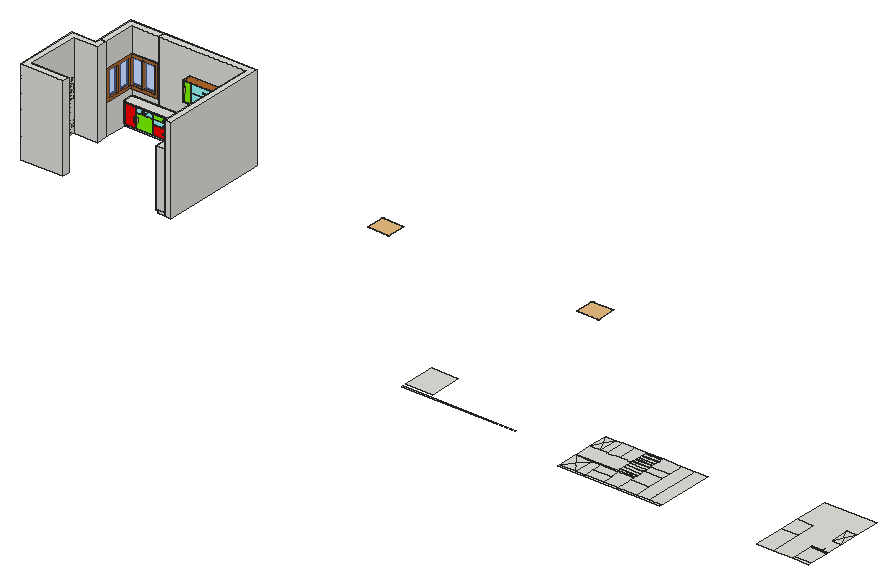
# SketchUp Ruby script. Lengths in millimetres.
U = 1.mm
M = Sketchup.active_model
def pt(a) = Geom::Point3d.new(a.map { |v| v * U })
def face(e, loops, mat)
  f = e.add_face(loops[0].map { |a| pt(a) })
  loops[1..].each { |l| e.add_face(l.map { |a| pt(a) }).erase! }
  f.material = f.back_material = mat if mat
  f
end
# faces: each face lists its corners as indices into pts; further lists are holes
def faces(e, pts, list, mat = nil) = list.each { |f| face(e, (f[0].is_a?(Array) ? f : [f]).map { |l| l.map { |i| pts[i] } }, mat) }
# xy, xz, yz: faces in a plane at the given z, y or x. An outline is a flat list of corners, or four numbers for a rectangle; further outlines are holes
def ring(l) = l.size == 4 ? [[l[0], l[1]], [l[2], l[1]], [l[2], l[3]], [l[0], l[3]]] : l.each_slice(2).to_a
def flat(e, list, mat, &to3) = list.each { |f| face(e, (f[0].is_a?(Array) ? f : [f]).map { |l| ring(l).map { |u, v| to3.(u, v) } }, mat) }
def xy(e, z, list, mat = nil) = flat(e, list, mat) { |x, y| [x, y, z] }
def xz(e, y, list, mat = nil) = flat(e, list, mat) { |x, z| [x, y, z] }
def yz(e, x, list, mat = nil) = flat(e, list, mat) { |y, z| [x, y, z] }
def lines(e, pts, list) = list.each { |a, b| e.add_line(pt(pts[a]), pt(pts[b])) }
# prism: a flat outline (further loops are holes) pulled along v
def prism(e, loops, v, mat = nil)
  f = face(e, loops, mat); d = Geom::Vector3d.new(v.map { |x| x * U })
  f.pushpull(f.normal.samedirection?(d) ? d.length : -d.length)
end
def box(e, o, s, mat = nil) = prism(e, [[o, [o[0] + s[0], o[1], o[2]], [o[0] + s[0], o[1] + s[1], o[2]], [o[0], o[1] + s[1], o[2]]]], [0, 0, s[2]], mat)
def at(x, y, z, deg = 0) = Geom::Transformation.translation(pt([x, y, z])) * Geom::Transformation.rotation(ORIGIN, Z_AXIS, deg.degrees)
def axes(o, x, y, z) = Geom::Transformation.new([*x, 0, *y, 0, *z, 0, *pt(o).to_a, 1])
def part(name) = M.definitions.add(name)
# library, detail: a bought-in or finely detailed component or shape, given as its bounding box
def library(name, o, s) = part(name).tap { |d| box(d.entities, o, s) }
def detail(e, o, s) = box(e.add_group.entities, o, s)
def put(e, d, t, mat = nil) = e.add_instance(d, t).tap { |i| i.material = mat if mat }
def group(e, t, mat = nil) = e.add_group.tap { |g| g.transformation = t; g.material = mat if mat }.entities
root = M.entities
M.materials.add("[Color A05]").color = [255, 0, 0]
M.materials.add("[Color F05]").color = [127, 255, 0]
M.materials.add("[Color H02]").color = [153, 255, 255]
M.materials.add("[Marble Carrara Floor Tile]").color = [204, 208, 219]
M.materials.add("[Marble Carrara Gold Floor Tile]").color = [225, 223, 217]
M.materials.add("[Translucent Glass Blue]").color = [100, 149, 237]
M.materials["[Translucent Glass Blue]"].alpha = 0.5
M.materials.add("[Wood Bamboo]").color = [177, 105, 43]
c1 = library("Range-Oven - 30 in top\#1",[-96,-83.2,0],[192,166.4,0.1])
c2 = library("6-POIGNEE CLC2",[-85,-7.5,0],[170,15,36])
c3 = library("1-POIGNEE CLC2\#1",[-77,-9.5,0],[154,19,36])
c4 = library("1-POIGNEE CLC2\#2",[-77,-9.5,0],[154,19,36])
c5 = library("1-POIGNEE CLC2\#3",[-77,-9.5,0],[154,19,36])
c6 = part("Group43\#2")
xy(c6.entities,0,[[-450.1,-460.6,-15,460.6],[15,-460.6,450.1,460.6]])
c7 = part("Group42\#1")
prism(c7.entities,[[[-550.1,560.6,0],[550.1,560.6,0],[550.1,-560.6,0],[-550.1,-560.6,0]],[[-15,-460.6,0],[-15,460.6,0],[-450.1,460.6,0],[-450.1,-460.6,0]],[[15,-460.6,0],[450.1,-460.6,0],[450.1,460.6,0],[15,460.6,0]]],[0,0,150])
put(c7.entities,c6,at(0,0,75),"[Translucent Glass Blue]")
c8 = part("Group45\#2")
xy(c8.entities,0,[[-489.5,-460.6,-15,460.6],[15,-460.6,489.5,460.6]])
c9 = part("Group44\#1")
prism(c9.entities,[[[589.5,-560.6,0],[-589.5,-560.6,0],[-589.5,560.6,0],[589.5,560.6,0]],[[-15,460.6,0],[-489.5,460.6,0],[-489.5,-460.6,0],[-15,-460.6,0]],[[489.5,-460.6,0],[489.5,460.6,0],[15,460.6,0],[15,-460.6,0]]],[0,0,150])
put(c9.entities,c8,at(0,0,75),"[Translucent Glass Blue]")
xy(root,0,[[16319,800,20369,840],[30877.5,840,31457.5,863.9],[16319,1000,17269,2140],[0,4244.1,0,6550.1,850,6550.1,850,6722.1,1078,6722.1,1078,6322.1,228,6322.1,228,4472.1,1528,4472.1,1528,4244.1],[5128,4244.1,5128,7862.1,2028,7862.1,2028,8090.1,5356,8090.1,5356,4244.1]])
xy(root,1488,[[3128,7562.1,5128,7862.1]],"[Wood Bamboo]")
xy(root,1524,[[3164,7562.1,3419,7844.1],[3437,7562.1,4519,7844.1],[4537,7562.1,4769,7844.1],[4787,7562.1,5092,7844.1]])
xy(root,1879,[[3437,7562.1,4519,7844.1]])
xy(root,1897,[[3437,7562.1,4519,7844.1]])
xy(root,2152,[[3164,7562.1,3419,7844.1],[3437,7562.1,4519,7844.1],[4537,7562.1,4769,7844.1],[4787,7562.1,4796,7844.1]])
xy(root,2152,[[4796,7562.1,5092,7844.1]],"[Wood Bamboo]")
xy(root,2188,[[3128,7562.1,5128,7862.1]],"[Wood Bamboo]")
xy(root,3048,[[0,4244.1,1528,4244.1,1528,4472.1,228,4472.1,228,6322.1,1078,6322.1,1078,6722.1,850,6722.1,850,6550.1,0,6550.1],[5128,4244.1,5356,4244.1,5356,8090.1,2028,8090.1,2028,7862.1,5128,7862.1]])
xz(root,4244.1,[[0,0,1528,3048],[5128,0,5356,3048]])
xz(root,4472.1,[[228,0,1528,3048]])
xz(root,6322.1,[[228,0,1078,3048]])
xz(root,6550.1,[[0,0,850,3048]])
xz(root,6722.1,[[850,0,1078,3048]])
xz(root,7562.1,[[[3128,1488,5128,1488,5092,1560,5092,1524,4787,1524,4787,2152,4796,2152,4778,2188,3128,2188],[3437,1524,4519,1879],[3437,1897,4519,2152],[3164,1524,3419,2152],[4537,1524,4769,2152]],[5128,1488,5128,2188,4778,2188,4796,2152,5092,2152,5092,1560],[4787,1524,5092,1560],[4787,1560,5092,2152]],"[Wood Bamboo]")
xz(root,7844.1,[[3164,1524,3419,2152],[3437,1524,4519,1879],[4537,1524,4769,2152],[4787,1524,5092,1560],[4787,1560,4787,2152,4796,2152,5092,1560],
  [5092,1560,4796,2152,5092,2152],[3437,1897,4519,2152]])
xz(root,7862.1,[[2028,0,5128,0,5128,1488,3128,1488,3128,2188,5128,2188,5128,3048,2028,3048]])
xz(root,8090.1,[[2028,0,5356,3048]])
yz(root,0,[[4244.1,0,6550.1,3048]])
yz(root,228,[[4472.1,0,5052.1,100],[5052.1,0,6322.1,0,6322.1,3048,4472.1,3048,4472.1,863.9,5052.1,863.9]])
yz(root,850,[[6550.1,0,6722.1,3048]])
yz(root,1078,[[6322.1,0,6722.1,3048]])
yz(root,1528,[[4244.1,0,4472.1,3048]])
yz(root,2028,[[7862.1,0,8090.1,3048]])
yz(root,3128,[[7562.1,1488,7862.1,2188]],"[Wood Bamboo]")
yz(root,3164,[[7562.1,1524,7844.1,2152]])
yz(root,3419,[[7562.1,1524,7844.1,2152]])
yz(root,3437,[[7562.1,1524,7844.1,1879],[7562.1,1897,7844.1,2152]])
yz(root,4519,[[7562.1,1524,7844.1,1879],[7562.1,1897,7844.1,2152]])
yz(root,4537,[[7562.1,1524,7844.1,2152]])
yz(root,4769,[[7562.1,1524,7844.1,2152]])
yz(root,4787,[[7562.1,1524,7844.1,2152]])
yz(root,5092,[[7562.1,1524,7844.1,2152]])
yz(root,5128,[[4244.1,0,4244.1,3048,7862.1,3048,7862.1,2188,7562.1,2188,7562.1,1488,7862.1,1488,7862.1,0]])
yz(root,5356,[[4244.1,0,8090.1,3048]])
# 1570 loose lines left out
put(root,c1,axes([17833.3,7531.9,0],[3.96989,0,0],[0,3.96989,0],[0,0,3.96989]))
put(root,c1,axes([10322.9,7603,0],[3.96989,0,0],[0,3.96989,0],[0,0,3.96989]))
put(root,c2,axes([1831.7,7481.1,712.4],[1,0,0],[0,0,1],[0,-1,0]))
put(root,c2,axes([2612.1,7481.1,712.4],[1,0,0],[0,0,1],[0,-1,0]))
put(root,c2,axes([3328,7481.1,712.4],[1,0,0],[0,0,1],[0,-1,0]))
put(root,c2,axes([2612.1,7481.1,517.4],[1,0,0],[0,0,1],[0,-1,0]))
put(root,c2,axes([2612.1,7481.1,277.4],[1,0,0],[0,0,1],[0,-1,0]))
put(root,c3,axes([1488.4,7481.1,388.6],[0,0,1],[-1,0,0],[0,-1,0]))
put(root,c3,axes([1586.7,7481.1,387.4],[0,0,1],[-1,0,0],[0,-1,0]))
put(root,c3,axes([3568.7,7481.1,387.4],[0,0,1],[-1,0,0],[0,-1,0]))
put(root,c3,axes([3703.7,7481.1,387.4],[0,0,1],[-1,0,0],[0,-1,0]))
put(root,c3,axes([4490.7,7481.1,387.4],[0,0,1],[-1,0,0],[0,-1,0]))
put(root,c3,axes([4610.7,7481.1,387.4],[0,0,1],[-1,0,0],[0,-1,0]))
put(root,c4,axes([3948.2,7544.1,1718.9],[1,0,0],[0,0,1],[0,-1,0]))
put(root,c4,axes([3948.2,7544.1,2025.9],[1,0,0],[0,0,1],[0,-1,0]))
put(root,c5,axes([3214.2,7544.1,1899],[0,0,1],[-1,0,0],[0,-1,0]))
put(root,c5,axes([4732.2,7544.1,1899],[0,0,1],[-1,0,0],[0,-1,0]))
g1 = group(root,at(850,6722.1,0))
prism(g1,[[[1178,1140,0],[228,1140,0],[228,0,0],[0,0,0],[0,1368,0],[1178,1368,0]]],[0,0,1066.8])
g2 = group(root,at(850,7849.1,0))
xy(g2,0,[[228,-300,4278,13]])
xy(g2,100,[[228,-350,678,-300],[678,-350,1278,-300],[1278,-350,2178,-300],[2178,-350,2778,-300],[2778,-350,3378,-300],
  [3378,-350,3698,-300],[3698,-350,4278,-300],[228,-300,678,0],[678,-300,1278,0],[1278,-300,2178,0],
  [2178,-300,2778,0],[2778,-300,3378,0],[3378,-300,3698,0],[3698,-300,4278,0],[228,0,678,13],
  [678,0,1278,13],[1278,0,2178,13],[2178,0,2778,13],[2778,0,3378,13],[3378,0,3698,13],
  [3698,0,4278,13]])
xy(g2,118,[[278,-350,669,0],[687,-350,1269,0],[1287,-350,2169,0],[2187,-350,2769,0],[2787,-350,3369,0],
  [3387,-350,3689,0],[3707,-350,4228,0]])
xy(g2,441,[[1287,-350,2169,0]])
xy(g2,459,[[1287,-350,2169,0]])
xy(g2,616,[[687,-350,1269,0],[1287,-350,2169,0],[2187,-350,2769,0]])
xy(g2,634,[[687,-350,1269,0],[1287,-350,2169,0],[2187,-350,2769,0]])
xy(g2,782,[[278,-350,669,0],[687,-350,1269,0],[1287,-350,2169,0],[2187,-350,2769,0],[2787,-350,3369,0],
  [3387,-350,3689,0],[3707,-350,4228,0]])
xy(g2,800,[[228,-350,4278,0]])
xz(g2,-350,[[[228,100,4278,800],[2787,118,3369,782],[3707,118,4228,782],[687,118,1269,616],[2187,118,2769,616],[1287,118,2169,441],[278,118,669,782],[3387,118,3689,782],[1287,459,2169,616],[1287,634,2169,782],[687,634,1269,782],[2187,634,2769,782]]],"[Wood Bamboo]")
xz(g2,-300,[[228,0,4278,100]],"[Marble Carrara Floor Tile]")
xz(g2,0,[[[228,100,4278,800],[2787,118,3369,782],[3707,118,4228,782],[687,118,1269,616],[2187,118,2769,616],[1287,118,2169,441],[278,118,669,782],[3387,118,3689,782],[1287,459,2169,616],[1287,634,2169,782],[687,634,1269,782],[2187,634,2769,782]],[278,118,669,782],[687,118,1269,616],[1287,118,2169,441],[2187,118,2769,616],
  [2787,118,3369,782],[3387,118,3689,782],[3707,118,4228,782],[1287,459,2169,616],[687,634,1269,782],
  [1287,634,2169,782],[2187,634,2769,782]])
xz(g2,13,[[228,0,4278,100]])
yz(g2,228,[[-300,0,13,100],[-350,100,0,800]])
yz(g2,278,[[-350,118,0,782]])
yz(g2,669,[[-350,118,0,625],[-350,625,0,782]])
yz(g2,687,[[-350,118,0,616],[-350,634,0,782]])
yz(g2,1269,[[-350,118,0,450],[-350,450,0,616],[-350,634,0,782]])
yz(g2,1287,[[-350,118,0,441],[-350,459,0,616],[-350,634,0,782]])
yz(g2,2169,[[-350,118,0,441],[-350,459,0,616],[-350,634,0,782]])
yz(g2,2187,[[-350,118,0,616],[-350,634,0,782]])
yz(g2,2769,[[-350,118,0,616],[-350,634,0,782]])
yz(g2,2787,[[-350,118,0,782]])
yz(g2,3369,[[-350,118,0,782]])
yz(g2,3387,[[-350,118,0,782]])
yz(g2,3689,[[-350,118,0,782]])
yz(g2,3707,[[-350,118,0,782]])
yz(g2,4228,[[-350,118,0,782]])
yz(g2,4278,[[-300,0,13,100],[-350,100,0,800]])
# 2 loose lines left out
g3 = group(g2,at(228,0,800),"[Marble Carrara Gold Floor Tile]")
xy(g3,0,[[20,-400,14.8,-399.3,10,-397.3,5.9,-394.1,2.7,-390,0.7,-385.2,0,-380,0,0,4050,0,4050,-400]])
xy(g3,40,[[0,-380,4050,0]])
xz(g3,-400,[[20,0,4050,20]])
xz(g3,0,[[0,0,4050,40]])
yz(g3,0,[[-380,0,0,40]])
yz(g3,4050,[[-400,0,0,0,0,40,-380,40,-385.2,39.3,-390,37.3,-394.1,34.1,-397.3,30,-399.3,25.2,-400,20]])
p = [[20,-400,0],[20,-400,20],[14.8,-399.3,25.2],[14.8,-399.3,0],[10,-397.3,30],[10,-397.3,0],
  [5.9,-394.1,34.1],[5.9,-394.1,0],[2.7,-390,37.3],[2.7,-390,0],[0.7,-385.2,39.3],[0.7,-385.2,0],
  [0,-380,40],[0,-380,0],[4050,-400,20],[4050,-399.3,25.2],[4050,-397.3,30],[4050,-394.1,34.1],
  [4050,-390,37.3],[4050,-385.2,39.3],[4050,-380,40]]
faces(g3,p,[[0,1,2,3],[3,2,4,5],[5,4,6,7],[7,6,8,9],[9,8,10,11],[11,10,12,13],[1,14,15,2],[2,15,16,4],
  [4,16,17,6],[6,17,18,8],[8,18,19,10],[10,19,20,12]])
g4 = group(root,at(1128,7499.1,118),"[Color A05]")
box(g4,[-3,-18,-3],[397,18,670])
g5 = group(root,at(1537,7499.1,634),"[Color H02]")
box(g5,[-3,-18,-3],[587,18,154])
g6 = group(root,at(1537,7499.1,118),"[Color F05]")
box(g6,[-3,-18,-3],[588,18,504])
g7 = group(root,at(2137,7499.1,634),"[Color F05]")
box(g7,[-3,-18,-3],[888,18,154])
g8 = group(root,at(2137,7499.1,459),"[Color H02]")
box(g8,[-3,-18,-3],[888,18,163])
g9 = group(root,at(2137,7499.1,118),"[Color A05]")
box(g9,[-3,-18,-3],[888,18,329])
g10 = group(root,at(3037,7499.1,634),"[Color A05]")
box(g10,[-3,-18,-3],[588,18,154])
g11 = group(root,at(3037,7499.1,118),"[Color H02]")
box(g11,[-3,-18,-3],[588,18,504])
g12 = group(root,at(3637,7499.1,118),"[Color F05]")
box(g12,[-3,-18,-3],[588,18,670])
g13 = group(root,at(4237,7499.1,118),"[Color H02]")
box(g13,[-3,-18,-3],[308,18,670])
g14 = group(root,at(4557,7499.1,118),"[Color A05]")
box(g14,[-3,-18,-3],[527,18,670])
g15 = group(root,at(850,6722.1,1981.2))
prism(g15,[[[1178,1140,206.8],[228,1140,206.8],[228,0,206.8],[0,0,206.8],[0,1368,206.8],[1178,1368,206.8]]],[0,0,860])
g16 = group(root,at(3164,7562.1,1524),"[Color F05]")
box(g16,[-3,-18,-3],[261,18,634])
g17 = group(root,at(3437,7562.1,1897),"[Color H02]")
box(g17,[-3,-18,-3],[1088,18,261])
g18 = group(root,at(3437,7562.1,1524),"[Color H02]")
box(g18,[-3,-18,-3],[1088,18,361])
g19 = group(root,at(4537,7562.1,1524),"[Color F05]")
box(g19,[-3,-18,-3],[238,18,634])
put(root,c7,axes([1477.9,7826.1,1627.4],[-1,0,0],[0,0,1],[0,1,0]),"[Wood Bamboo]")
put(root,c9,axes([1077.9,7311.6,1627.4],[0,-1,0],[0,0,1],[-1,0,0]),"[Wood Bamboo]")
g20 = group(root,at(22519.6,0,0))
xy(g20,0,[[0,0,3618,100],[0,100,290,450,0,800],[0,100,580,100,290,450],[580,100,580,800,290,450],[580,100,900,800],
  [900,100,1550,450],[1550,100,2068,800],[2068,100,2718,666],[2718,100,3168,2140],[3168,100,3618,2140],
  [290,450,580,800,0,800],[900,450,1550,800],[2068,666,2718,1266],[0,800,2068,840],[0,840,1468,1440],
  [1468,840,2068,948],[1468,948,2068,968],[1468,968,2068,1094.4],[1468,1094.4,2068,1114.4],[1468,1114.4,2068,1222.4],
  [1468,1222.4,2068,1242.4],[1468,1242.4,2068,1368.8],[2068,1266,2718,1574],[1468,1368.8,2068,1388.8],[1468,1388.8,2068,1496.8],
  [0,1440,175,1790,0,2140],[0,1440,350,1440,175,1790],[350,1440,350,2140,175,1790],[350,1440,600,2140],[600,1440,1025,2140],
  [1025,1440,1450,2140],[1450,1440,1468,2140],[1468,1496.8,2068,1516.8],[1468,1516.8,2068,1643.2],[2068,1574,2718,2140],
  [1468,1643.2,2068,1663.2],[1468,1663.2,2068,1771.2],[1468,1771.2,2068,1791.2],[175,1790,350,2140,0,2140],[1468,1791.2,2068,1917.6],
  [1468,1917.6,2068,1937.6],[1468,1937.6,2068,2065.8],[1468,2065.8,2068,2085.8],[1468,2085.8,2068,2140]])
# 3 loose lines left out
g21 = group(root,at(5128,7862.1,0))
xy(g21,0,[[-250,-3618,0,-580]])
xy(g21,100,[[-300,-3618,-250,-580]])
xy(g21,136,[[-300,-3600,0,-3177],[-300,-3159,0,-2727],[-300,-2709,0,-2077],[-300,-2059,0,-1559],[-300,-1541,0,-909],
  [-300,-891,0,-598]])
xy(g21,441,[[-300,-1541,0,-909]])
xy(g21,459,[[-300,-1541,0,-909]])
xy(g21,657,[[-300,-2709,0,-2077]])
xy(g21,675,[[-300,-2709,0,-2077]])
xy(g21,800,[[-300,-1559,0,-1541],[-300,-909,0,-891],[-300,-598,0,-580]])
xy(g21,1257,[[-300,-2709,0,-2077]])
xy(g21,1275,[[-300,-2709,0,-2077]])
xy(g21,1440,[[-300,-1468,0,-341]])
xy(g21,1458,[[-300,-1450,0,-1034],[-300,-1016,0,-609],[-300,-591,0,-359]])
xy(g21,1565,[[-300,-2709,0,-2077]])
xy(g21,1583,[[-300,-2709,0,-2077]])
xy(g21,2104,[[-300,-3600,0,-3177],[-300,-3159,0,-2727],[-300,-2709,0,-2077],[-300,-2059,0,-1468],[-300,-1450,0,-1034],
  [-300,-1016,0,-609],[-300,-591,0,-359]])
xy(g21,2140,[[-300,-3618,0,-341]])
xz(g21,-3618,[[-250,0,0,100],[-300,100,0,2140]])
xz(g21,-3600,[[-300,136,0,2104]])
xz(g21,-3177,[[-300,136,0,2104]])
xz(g21,-3159,[[-300,136,0,2104]])
xz(g21,-2727,[[-300,136,0,2104]])
xz(g21,-2709,[[-300,136,0,657],[-300,675,0,1257],[-300,1275,0,1565],[-300,1583,0,2104]])
xz(g21,-2077,[[-300,136,0,657],[-300,675,0,1257],[-300,1275,0,1565],[-300,1583,0,2104]])
xz(g21,-2059,[[-300,136,0,800],[-300,800,0,840],[-300,840,0,2104]])
xz(g21,-1559,[[-300,136,0,800]])
xz(g21,-1541,[[-300,136,0,441],[-300,459,0,800]])
xz(g21,-1468,[[-300,1440,0,2104]])
xz(g21,-1450,[[-300,1458,0,2104]])
xz(g21,-1034,[[-300,1458,0,2104]])
xz(g21,-1016,[[-300,1458,0,2104]])
xz(g21,-909,[[-300,136,0,441],[-300,459,0,800]])
xz(g21,-891,[[-300,136,0,800]])
xz(g21,-609,[[-300,1458,0,2104]])
xz(g21,-598,[[-300,136,0,800]])
xz(g21,-591,[[-300,1458,0,2104]])
xz(g21,-580,[[-250,0,0,100],[-300,100,0,800]])
xz(g21,-359,[[-300,1458,0,2104]])
xz(g21,-341,[[-300,1440,0,2140]])
yz(g21,-300,[[[-3618,100,-3618,2140,-341,2140,-341,1440,-1468,1440,-1468,2104,-2059,2104,-2059,136,-1559,136,-1559,800,-1541,800,-1541,459,-909,459,-909,800,-891,800,-891,136,-598,136,-598,800,-580,800,-580,100],[-3159,136,-2727,2104],[-3600,136,-3177,2104],[-2709,675,-2077,1257],[-2709,136,-2077,657],[-2709,1583,-2077,2104],[-1450,1458,-1034,2104],[-1016,1458,-609,2104],[-1541,136,-909,441],[-2709,1275,-2077,1565],[-591,1458,-359,2104]]])
yz(g21,-250,[[-3618,0,-580,100]])
yz(g21,0,[[-3600,136,-3177,2104],[-3159,136,-2727,2104],[-2709,136,-2077,657],[-2059,136,-1559,800],[-1541,136,-909,441],
  [-891,136,-598,800],[-1541,459,-909,800],[-2709,675,-2077,1257],[-2059,840,-1468,2104],[-2709,1275,-2077,1565],
  [-1450,1458,-1034,2104],[-1016,1458,-609,2104],[-591,1458,-359,2104],[-2709,1583,-2077,2104]])
g22 = group(g21,at(0,-580,800))
xy(g22,0,[[-330,-1479,0,-979],[-330,-979,0,-961],[-330,-961,0,-329],[-330,-329,0,-311],[-330,-311,0,-18],
  [-330,-18,0,0]])
xy(g22,40,[[-330,-1479,0,0]])
xz(g22,-1479,[[-330,0,0,40]])
xz(g22,0,[[-330,0,-335.2,0.7,-340,2.7,-344.1,5.9,-347.3,10,-349.3,14.8,-350,20,-349.3,25.2,-347.3,30,-344.1,34.1,-340,37.3,-335.2,39.3,-330,40,0,40,0,0]])
yz(g22,0,[[-1479,0,0,40]])
p = [[-335.2,-1478.3,0.7],[-335.2,-979,0.7],[-330,-979,0],[-330,-1479,0],[-335.2,-1478.3,39.3],[-330,-1479,40],
  [-335.2,-961,0.7],[-330,-961,0],[-335.2,-329,0.7],[-330,-329,0],[-335.2,-311,0.7],[-330,-311,0],
  [-335.2,-18,0.7],[-330,-18,0],[-335.2,0,0.7],[-330,0,0],[-340,-1476.3,2.7],[-340,-979,2.7],
  [-340,-1476.3,37.3],[-340,-961,2.7],[-340,-329,2.7],[-340,-311,2.7],[-340,-18,2.7],[-340,0,2.7],
  [-344.1,-1473.1,5.9],[-344.1,-979,5.9],[-344.1,-1473.1,34.1],[-344.1,-961,5.9],[-344.1,-329,5.9],[-344.1,-311,5.9],
  [-344.1,-18,5.9],[-344.1,0,5.9],[-347.3,-1469,10],[-347.3,-979,10],[-347.3,-1469,30],[-347.3,-961,10],
  [-347.3,-329,10],[-347.3,-311,10],[-347.3,-18,10],[-347.3,0,10],[-349.3,-1464.2,14.8],[-349.3,-979,14.8],
  [-349.3,-1464.2,25.2],[-349.3,-961,14.8],[-349.3,-329,14.8],[-349.3,-311,14.8],[-349.3,-18,14.8],[-349.3,0,14.8],
  [-350,-1459,20],[-350,-979,20],[-350,-961,20],[-350,-329,20],[-350,-311,20],[-350,-18,20],
  [-350,0,20],[-349.3,0,25.2],[-347.3,0,30],[-344.1,0,34.1],[-340,0,37.3],[-335.2,0,39.3],
  [-330,0,40]]
faces(g22,p,[[0,1,2,3],[4,0,3,5],[1,6,7,2],[6,8,9,7],[8,10,11,9],[10,12,13,11],[12,14,15,13],[16,17,1,0],
  [18,16,0,4],[17,19,6,1],[19,20,8,6],[20,21,10,8],[21,22,12,10],[22,23,14,12],[24,25,17,16],[26,24,16,18],
  [25,27,19,17],[27,28,20,19],[28,29,21,20],[29,30,22,21],[30,31,23,22],[32,33,25,24],[34,32,24,26],[33,35,27,25],
  [35,36,28,27],[36,37,29,28],[37,38,30,29],[38,39,31,30],[40,41,33,32],[42,40,32,34],[41,43,35,33],[43,44,36,35],
  [44,45,37,36],[45,46,38,37],[46,47,39,38],[48,49,41,40],[42,48,40],[49,50,43,41],[50,51,44,43],[51,52,45,44],
  [52,53,46,45],[53,54,47,46],[53,52,51,50,49,48,42,55,54],[55,42,34,56],[56,34,26,57],[57,26,18,58],[58,18,4,59],[59,4,5,60]])
g23 = group(root,at(29607.5,0,0))
xy(g23,0,[[0,0,600,1115.6],[600,0,1270,0,1270,863.9,1630,863.9,1630,1021.1,1585.9,1021.1,1585.9,983.5,1571.9,983.5,1571.9,1021.1,1541.8,1021.1,1541.8,1039.4,1651.5,1039.4,1651.5,863.9,1850,863.9,1850,1440,1500,1440,1500,2140,1850,2140,1850,3000,0,3000,0,1800,600,1800],[1270,0,1850,100],[1270,100,1850,800],[1270,800,1850,840],
  [0,1115.6,600,1800],[1500,1440,1675,1790,1500,2140],[1500,1440,1850,1440,1675,1790],[1850,1440,1850,2140,1675,1790],[1675,1790,1850,2140,1500,2140]])
g24 = group(root,at(228,4472.1,0))
box(g24,[0,0,0],[350,580,100])
g25 = group(root,at(228,4472.1,100))
box(g25,[0,0,0],[350,580,763.9])
g26 = group(root,at(228,6322.1,0))
yz(g26,0,[[-1850,0,-1270,100],[-600,0,0,1115.6],[-1850,100,-1270,800],[-1850,800,-1270,840],[-600,1115.6,0,1800]])
# 7 loose lines left out
